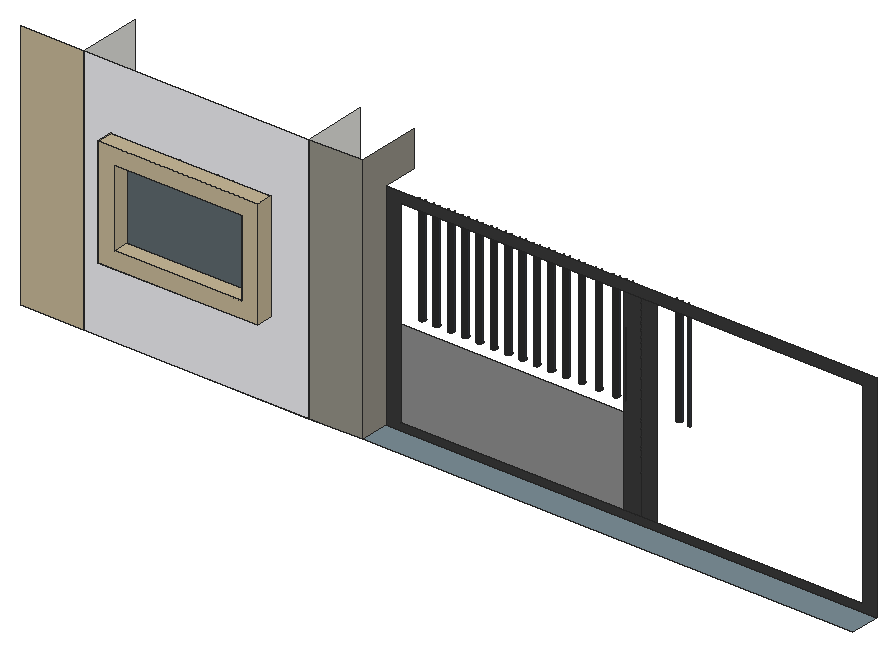
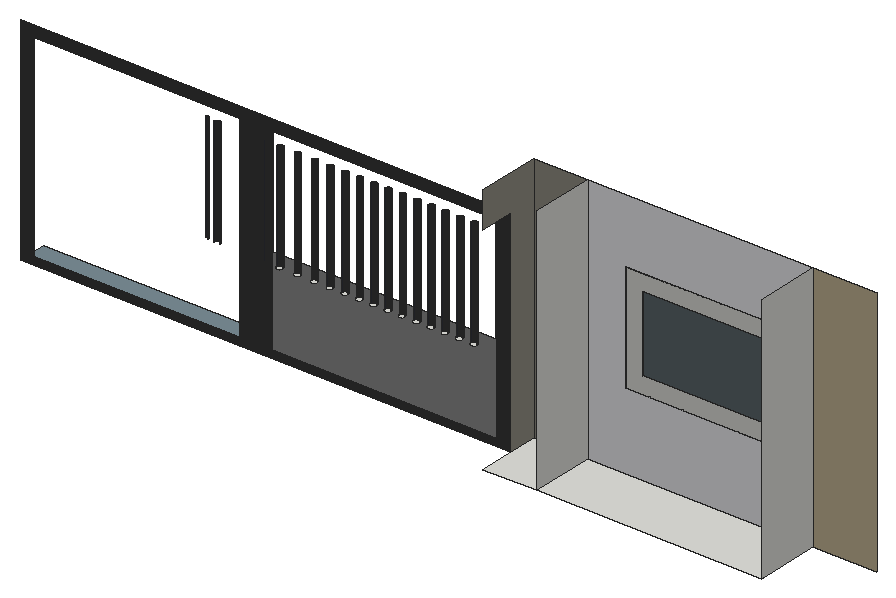
# SketchUp Ruby script. Lengths in inches.
U = 1.inch
M = Sketchup.active_model
def pt(a) = Geom::Point3d.new(a.map { |v| v * U })
def face(e, loops, mat)
  f = e.add_face(loops[0].map { |a| pt(a) })
  loops[1..].each { |l| e.add_face(l.map { |a| pt(a) }).erase! }
  f.material = f.back_material = mat if mat
  f
end
# faces: each face lists its corners as indices into pts; further lists are holes
def faces(e, pts, list, mat = nil) = list.each { |f| face(e, (f[0].is_a?(Array) ? f : [f]).map { |l| l.map { |i| pts[i] } }, mat) }
# xy, xz, yz: faces in a plane at the given z, y or x. An outline is a flat list of corners, or four numbers for a rectangle; further outlines are holes
def ring(l) = l.size == 4 ? [[l[0], l[1]], [l[2], l[1]], [l[2], l[3]], [l[0], l[3]]] : l.each_slice(2).to_a
def flat(e, list, mat, &to3) = list.each { |f| face(e, (f[0].is_a?(Array) ? f : [f]).map { |l| ring(l).map { |u, v| to3.(u, v) } }, mat) }
def xy(e, z, list, mat = nil) = flat(e, list, mat) { |x, y| [x, y, z] }
def xz(e, y, list, mat = nil) = flat(e, list, mat) { |x, z| [x, y, z] }
def yz(e, x, list, mat = nil) = flat(e, list, mat) { |y, z| [x, y, z] }
def lines(e, pts, list) = list.each { |a, b| e.add_line(pt(pts[a]), pt(pts[b])) }
# prism: a flat outline (further loops are holes) pulled along v
def prism(e, loops, v, mat = nil)
  f = face(e, loops, mat); d = Geom::Vector3d.new(v.map { |x| x * U })
  f.pushpull(f.normal.samedirection?(d) ? d.length : -d.length)
end
def box(e, o, s, mat = nil) = prism(e, [[o, [o[0] + s[0], o[1], o[2]], [o[0] + s[0], o[1] + s[1], o[2]], [o[0], o[1] + s[1], o[2]]]], [0, 0, s[2]], mat)
def at(x, y, z, deg = 0) = Geom::Transformation.translation(pt([x, y, z])) * Geom::Transformation.rotation(ORIGIN, Z_AXIS, deg.degrees)
def axes(o, x, y, z) = Geom::Transformation.new([*x, 0, *y, 0, *z, 0, *pt(o).to_a, 1])
def part(name) = M.definitions.add(name)
# library, detail: a bought-in or finely detailed component or shape, given as its bounding box
def library(name, o, s) = part(name).tap { |d| box(d.entities, o, s) }
def detail(e, o, s) = box(e.add_group.entities, o, s)
def put(e, d, t, mat = nil) = e.add_instance(d, t).tap { |i| i.material = mat if mat }
def group(e, t, mat = nil) = e.add_group.tap { |g| g.transformation = t; g.material = mat if mat }.entities
root = M.entities
M.materials.add("[Blinds Vertical Pattern]1").color = [239, 239, 242]
M.materials.add("[Color M04]").color = [142, 142, 142]
M.materials.add("[Color M07]").color = [58, 58, 58]
M.materials.add("[Formica Graystone]").color = [149, 146, 135]
M.materials.add("[Formica Laminate Dark]").color = [50, 53, 60]
M.materials.add("[Formica Speckled Grey]").color = [94, 105, 111]
M.materials.add("[Quartz Light Brown]").color = [199, 184, 152]
M.materials.add("[Square Glass Tile 01]").color = [123, 142, 151]
xy(root,0,[[14.76,96.24,66.82,111],[66.82,96.24,79.1,111]])
xy(root,0,[[79.1,96.24,192.64,102.91]],"[Square Glass Tile 01]")
xy(root,17.84,[[20.96,92.55,57.83,96.24]],"[Quartz Light Brown]")
xy(root,21.59,[[24.71,92.55,54.08,96.24]],"[Quartz Light Brown]")
xy(root,22.1875,[[84.71,106,84.53,106.02,84.36,106.09,84.22,106.2,84.11,106.34,84.04,106.51,84.02,106.6875,84.04,106.87,84.11,107.03,84.22,107.17,84.36,107.28,84.53,107.35,84.71,107.375,84.89,107.35,85.05,107.28,85.19,107.17,85.3,107.03,85.37,106.87,85.4,106.6875,85.37,106.51,85.3,106.34,85.19,106.2,85.05,106.09,84.89,106.02],[88.02,106,87.84,106.02,87.68,106.09,87.53,106.2,87.42,106.34,87.36,106.51,87.33,106.6875,87.36,106.87,87.42,107.03,87.53,107.17,87.68,107.28,87.84,107.35,88.02,107.375,88.2,107.35,88.36,107.28,88.51,107.17,88.62,107.03,88.68,106.87,88.71,106.6875,88.68,106.51,88.62,106.34,88.51,106.2,88.36,106.09,88.2,106.02],[91.33,106,91.15,106.02,90.99,106.09,90.85,106.2,90.74,106.34,90.67,106.51,90.65,106.6875,90.67,106.87,90.74,107.03,90.85,107.17,90.99,107.28,91.15,107.35,91.33,107.375,91.51,107.35,91.68,107.28,91.82,107.17,91.93,107.03,92,106.87,92.02,106.6875,92,106.51,91.93,106.34,91.82,106.2,91.68,106.09,91.51,106.02],[94.65,106,94.47,106.02,94.3,106.09,94.16,106.2,94.05,106.34,93.98,106.51,93.96,106.6875,93.98,106.87,94.05,107.03,94.16,107.17,94.3,107.28,94.47,107.35,94.65,107.375,94.82,107.35,94.99,107.28,95.13,107.17,95.24,107.03,95.31,106.87,95.33,106.6875,95.31,106.51,95.24,106.34,95.13,106.2,94.99,106.09,94.82,106.02],[97.96,106,97.78,106.02,97.61,106.09,97.47,106.2,97.36,106.34,97.29,106.51,97.27,106.6875,97.29,106.87,97.36,107.03,97.47,107.17,97.61,107.28,97.78,107.35,97.96,107.375,98.14,107.35,98.3,107.28,98.44,107.17,98.55,107.03,98.62,106.87,98.65,106.6875,98.62,106.51,98.55,106.34,98.44,106.2,98.3,106.09,98.14,106.02],
  [101.27,106,101.09,106.02,100.93,106.09,100.78,106.2,100.67,106.34,100.61,106.51,100.58,106.6875,100.61,106.87,100.67,107.03,100.78,107.17,100.93,107.28,101.09,107.35,101.27,107.375,101.45,107.35,101.61,107.28,101.76,107.17,101.87,107.03,101.93,106.87,101.96,106.6875,101.93,106.51,101.87,106.34,101.76,106.2,101.61,106.09,101.45,106.02],[104.58,106,104.4,106.02,104.24,106.09,104.1,106.2,103.99,106.34,103.92,106.51,103.9,106.6875,103.92,106.87,103.99,107.03,104.1,107.17,104.24,107.28,104.4,107.35,104.58,107.375,104.76,107.35,104.93,107.28,105.07,107.17,105.18,107.03,105.25,106.87,105.27,106.6875,105.25,106.51,105.18,106.34,105.07,106.2,104.93,106.09,104.76,106.02],[107.9,106,107.72,106.02,107.55,106.09,107.41,106.2,107.3,106.34,107.23,106.51,107.21,106.6875,107.23,106.87,107.3,107.03,107.41,107.17,107.55,107.28,107.72,107.35,107.9,107.375,108.07,107.35,108.24,107.28,108.38,107.17,108.49,107.03,108.56,106.87,108.58,106.6875,108.56,106.51,108.49,106.34,108.38,106.2,108.24,106.09,108.07,106.02],[111.21,106,111.03,106.02,110.86,106.09,110.72,106.2,110.61,106.34,110.54,106.51,110.52,106.6875,110.54,106.87,110.61,107.03,110.72,107.17,110.86,107.28,111.03,107.35,111.21,107.375,111.39,107.35,111.55,107.28,111.69,107.17,111.8,107.03,111.87,106.87,111.9,106.6875,111.87,106.51,111.8,106.34,111.69,106.2,111.55,106.09,111.39,106.02],[114.52,106,114.34,106.02,114.18,106.09,114.03,106.2,113.92,106.34,113.86,106.51,113.83,106.6875,113.86,106.87,113.92,107.03,114.03,107.17,114.18,107.28,114.34,107.35,114.52,107.375,114.7,107.35,114.86,107.28,115.01,107.17,115.12,107.03,115.18,106.87,115.21,106.6875,115.18,106.51,115.12,106.34,115.01,106.2,114.86,106.09,114.7,106.02],
  [117.96,106,117.78,106.02,117.61,106.09,117.47,106.2,117.36,106.34,117.29,106.51,117.27,106.6875,117.29,106.87,117.36,107.03,117.47,107.17,117.61,107.28,117.78,107.35,117.96,107.375,118.14,107.35,118.3,107.28,118.44,107.17,118.55,107.03,118.62,106.87,118.65,106.6875,118.62,106.51,118.55,106.34,118.44,106.2,118.3,106.09,118.14,106.02],[121.58,106,121.4,106.02,121.24,106.09,121.1,106.2,120.99,106.34,120.92,106.51,120.9,106.6875,120.92,106.87,120.99,107.03,121.1,107.17,121.24,107.28,121.4,107.35,121.58,107.375,121.76,107.35,121.93,107.28,122.07,107.17,122.18,107.03,122.25,106.87,122.27,106.6875,122.25,106.51,122.18,106.34,122.07,106.2,121.93,106.09,121.76,106.02],[125.52,106,125.34,106.02,125.18,106.09,125.03,106.2,124.92,106.34,124.86,106.51,124.83,106.6875,124.86,106.87,124.92,107.03,125.03,107.17,125.18,107.28,125.34,107.35,125.52,107.375,125.7,107.35,125.86,107.28,126.01,107.17,126.12,107.03,126.18,106.87,126.21,106.6875,126.18,106.51,126.12,106.34,126.01,106.2,125.86,106.09,125.7,106.02],[129.58,106,129.4,106.02,129.24,106.09,129.1,106.2,128.99,106.34,128.92,106.51,128.9,106.6875,128.92,106.87,128.99,107.03,129.1,107.17,129.24,107.28,129.4,107.35,129.58,107.375,129.76,107.35,129.93,107.28,130.07,107.17,130.18,107.03,130.25,106.87,130.27,106.6875,130.25,106.51,130.18,106.34,130.07,106.2,129.93,106.09,129.76,106.02]])
xy(root,39.28,[[24.71,92.55,54.08,96.24]],"[Quartz Light Brown]")
xy(root,43.03,[[20.96,92.55,57.83,96.24]],"[Quartz Light Brown]")
xz(root,92.55,[[[20.96,17.84,57.83,43.03],[24.71,21.59,54.08,39.28]]],"[Quartz Light Brown]")
xz(root,96.24,[[[20.96,17.84,57.83,43.03],[24.71,21.59,54.08,39.28]]])
xz(root,96.24,[[[14.76,0,66.82,57.8125],[20.96,17.84,57.83,43.03]]],"[Blinds Vertical Pattern]1")
xz(root,96.24,[[66.82,0,79.1,57.8125]],"[Formica Graystone]")
xz(root,96.24,[[24.71,21.59,54.08,39.28]],"[Formica Speckled Grey]")
xz(root,96.24,[[0,0,14.76,57.8125]],"[Quartz Light Brown]")
xz(root,102.91,[[82.65,1.75,134.27,22.1875]],"[Color M04]")
xz(root,102.91,[[[79.1,0,192.64,49.625],[82.65,1.75,189.5,47.21]],[134.27,1.75,138.0625,47.21],[138.0625,1.75,141.86,47.21]],"[Color M07]")
yz(root,14.76,[[96.24,0,111,57.8125]])
yz(root,20.96,[[92.55,17.84,96.24,43.03]],"[Quartz Light Brown]")
yz(root,24.71,[[92.55,21.59,96.24,39.28]],"[Quartz Light Brown]")
yz(root,54.08,[[92.55,21.59,96.24,39.28]],"[Quartz Light Brown]")
yz(root,57.83,[[92.55,17.84,96.24,43.03]],"[Quartz Light Brown]")
yz(root,66.82,[[96.24,0,111,57.8125]])
yz(root,79.1,[[96.24,0,102.91,0,102.91,49.625,111,49.625,111,57.8125,96.24,57.8125]],"[Formica Graystone]")
p = [[84.36,106.09,22.1875],[84.53,106.02,22.1875],[84.53,106.02,47.21],[84.36,106.09,47.21],[84.71,106,22.1875],[84.71,106,47.21],
  [84.89,106.02,22.1875],[84.89,106.02,47.21],[85.05,106.09,22.1875],[85.05,106.09,47.21],[87.68,106.09,22.1875],[87.84,106.02,22.1875],
  [87.84,106.02,47.21],[87.68,106.09,47.21],[88.02,106,22.1875],[88.02,106,47.21],[88.2,106.02,22.1875],[88.2,106.02,47.21],
  [88.36,106.09,22.1875],[88.36,106.09,47.21],[90.99,106.09,22.1875],[91.15,106.02,22.1875],[91.15,106.02,47.21],[90.99,106.09,47.21],
  [91.33,106,22.1875],[91.33,106,47.21],[91.51,106.02,22.1875],[91.51,106.02,47.21],[91.68,106.09,22.1875],[91.68,106.09,47.21],
  [94.3,106.09,22.1875],[94.47,106.02,22.1875],[94.47,106.02,47.21],[94.3,106.09,47.21],[94.65,106,22.1875],[94.65,106,47.21],
  [94.82,106.02,22.1875],[94.82,106.02,47.21],[94.99,106.09,22.1875],[94.99,106.09,47.21],[97.61,106.09,22.1875],[97.78,106.02,22.1875],
  [97.78,106.02,47.21],[97.61,106.09,47.21],[97.96,106,22.1875],[97.96,106,47.21],[98.14,106.02,22.1875],[98.14,106.02,47.21],
  [98.3,106.09,22.1875],[98.3,106.09,47.21],[100.93,106.09,22.1875],[101.09,106.02,22.1875],[101.09,106.02,47.21],[100.93,106.09,47.21],
  [101.27,106,22.1875],[101.27,106,47.21],[101.45,106.02,22.1875],[101.45,106.02,47.21],[101.61,106.09,22.1875],[101.61,106.09,47.21],
  [104.24,106.09,22.1875],[104.4,106.02,22.1875],[104.4,106.02,47.21],[104.24,106.09,47.21],[104.58,106,22.1875],[104.58,106,47.21],
  [104.76,106.02,22.1875],[104.76,106.02,47.21],[104.93,106.09,22.1875],[104.93,106.09,47.21],[107.55,106.09,22.1875],[107.72,106.02,22.1875],
  [107.72,106.02,47.21],[107.55,106.09,47.21],[107.9,106,22.1875],[107.9,106,47.21],[108.07,106.02,22.1875],[108.07,106.02,47.21],
  [108.24,106.09,22.1875],[108.24,106.09,47.21],[110.86,106.09,22.1875],[111.03,106.02,22.1875],[111.03,106.02,47.21],[110.86,106.09,47.21],
  [111.21,106,22.1875],[111.21,106,47.21],[111.39,106.02,22.1875],[111.39,106.02,47.21],[111.55,106.09,22.1875],[111.55,106.09,47.21],
  [114.18,106.09,22.1875],[114.34,106.02,22.1875],[114.34,106.02,47.21],[114.18,106.09,47.21],[114.52,106,22.1875],[114.52,106,47.21],
  [114.7,106.02,22.1875],[114.7,106.02,47.21],[114.86,106.09,22.1875],[114.86,106.09,47.21],[117.61,106.09,22.1875],[117.78,106.02,22.1875],
  [117.78,106.02,47.21],[117.61,106.09,47.21],[117.96,106,22.1875],[117.96,106,47.21],[118.14,106.02,22.1875],[118.14,106.02,47.21],
  [118.3,106.09,22.1875],[118.3,106.09,47.21],[121.24,106.09,22.1875],[121.4,106.02,22.1875],[121.4,106.02,47.21],[121.24,106.09,47.21],
  [121.58,106,22.1875],[121.58,106,47.21],[121.76,106.02,22.1875],[121.76,106.02,47.21],[121.93,106.09,22.1875],[121.93,106.09,47.21],
  [125.18,106.09,22.1875],[125.34,106.02,22.1875],[125.34,106.02,47.21],[125.18,106.09,47.21],[125.52,106,22.1875],[125.52,106,47.21],
  [125.7,106.02,22.1875],[125.7,106.02,47.21],[125.86,106.09,22.1875],[125.86,106.09,47.21],[129.24,106.09,22.1875],[129.4,106.02,22.1875],
  [129.4,106.02,47.21],[129.24,106.09,47.21],[129.58,106,22.1875],[129.58,106,47.21],[129.76,106.02,22.1875],[129.76,106.02,47.21],
  [129.93,106.09,22.1875],[129.93,106.09,47.21],[132.24,106.09,22.1875],[132.4,106.02,22.1875],[132.4,106.02,47.21],[132.24,106.09,47.21],
  [132.58,106,22.1875],[132.58,106,47.21],[132.76,106.02,22.1875],[132.76,106.02,47.21],[132.93,106.09,22.1875],[132.93,106.09,47.21],
  [143.74,106.09,22.1875],[143.9,106.02,22.1875],[143.9,106.02,47.21],[143.74,106.09,47.21],[144.08,106,22.1875],[144.08,106,47.21],
  [144.26,106.02,22.1875],[144.26,106.02,47.21],[144.43,106.09,22.1875],[144.43,106.09,47.21],[146.61,106.09,22.1875],[146.78,106.02,22.1875],
  [146.78,106.02,47.21],[146.61,106.09,47.21],[146.96,106,22.1875],[146.96,106,47.21],[147.14,106.02,22.1875],[147.14,106.02,47.21],
  [84.22,106.2,22.1875],[84.22,106.2,47.21],[85.19,106.2,22.1875],[85.19,106.2,47.21],[87.53,106.2,22.1875],[87.53,106.2,47.21],
  [88.51,106.2,22.1875],[88.51,106.2,47.21],[90.85,106.2,22.1875],[90.85,106.2,47.21],[91.82,106.2,22.1875],[91.82,106.2,47.21],
  [94.16,106.2,22.1875],[94.16,106.2,47.21],[95.13,106.2,22.1875],[95.13,106.2,47.21],[97.47,106.2,22.1875],[97.47,106.2,47.21],
  [98.44,106.2,22.1875],[98.44,106.2,47.21],[100.78,106.2,22.1875],[100.78,106.2,47.21],[101.76,106.2,22.1875],[101.76,106.2,47.21],
  [104.1,106.2,22.1875],[104.1,106.2,47.21],[105.07,106.2,22.1875],[105.07,106.2,47.21],[107.41,106.2,22.1875],[107.41,106.2,47.21],
  [108.38,106.2,22.1875],[108.38,106.2,47.21],[110.72,106.2,22.1875],[110.72,106.2,47.21],[111.69,106.2,22.1875],[111.69,106.2,47.21],
  [114.03,106.2,22.1875],[114.03,106.2,47.21],[115.01,106.2,22.1875],[115.01,106.2,47.21],[117.47,106.2,22.1875],[117.47,106.2,47.21],
  [118.44,106.2,22.1875],[118.44,106.2,47.21],[121.1,106.2,22.1875],[121.1,106.2,47.21],[122.07,106.2,22.1875],[122.07,106.2,47.21],
  [125.03,106.2,22.1875],[125.03,106.2,47.21],[126.01,106.2,22.1875],[126.01,106.2,47.21],[129.1,106.2,22.1875],[129.1,106.2,47.21],
  [130.07,106.2,22.1875],[130.07,106.2,47.21],[132.1,106.2,22.1875],[132.1,106.2,47.21],[133.07,106.2,22.1875],[133.07,106.2,47.21],
  [143.6,106.2,22.1875],[143.6,106.2,47.21],[144.57,106.2,22.1875],[144.57,106.2,47.21],[146.47,106.2,22.1875],[146.47,106.2,47.21],
  [84.11,106.34,22.1875],[84.11,106.34,47.21],[85.3,106.34,22.1875],[85.3,106.34,47.21],[87.42,106.34,22.1875],[87.42,106.34,47.21],
  [88.62,106.34,22.1875],[88.62,106.34,47.21],[90.74,106.34,22.1875],[90.74,106.34,47.21],[91.93,106.34,22.1875],[91.93,106.34,47.21],
  [94.05,106.34,22.1875],[94.05,106.34,47.21],[95.24,106.34,22.1875],[95.24,106.34,47.21],[97.36,106.34,22.1875],[97.36,106.34,47.21],
  [98.55,106.34,22.1875],[98.55,106.34,47.21],[100.67,106.34,22.1875],[100.67,106.34,47.21],[101.87,106.34,22.1875],[101.87,106.34,47.21],
  [103.99,106.34,22.1875],[103.99,106.34,47.21],[105.18,106.34,22.1875],[105.18,106.34,47.21],[107.3,106.34,22.1875],[107.3,106.34,47.21],
  [108.49,106.34,22.1875],[108.49,106.34,47.21],[110.61,106.34,22.1875],[110.61,106.34,47.21],[111.8,106.34,22.1875],[111.8,106.34,47.21],
  [113.92,106.34,22.1875],[113.92,106.34,47.21],[115.12,106.34,22.1875],[115.12,106.34,47.21],[117.36,106.34,22.1875],[117.36,106.34,47.21],
  [118.55,106.34,22.1875],[118.55,106.34,47.21],[120.99,106.34,22.1875],[120.99,106.34,47.21],[122.18,106.34,22.1875],[122.18,106.34,47.21],
  [124.92,106.34,22.1875],[124.92,106.34,47.21],[126.12,106.34,22.1875],[126.12,106.34,47.21],[128.99,106.34,22.1875],[128.99,106.34,47.21],
  [130.18,106.34,22.1875],[130.18,106.34,47.21],[131.99,106.34,22.1875],[131.99,106.34,47.21],[133.18,106.34,22.1875],[133.18,106.34,47.21],
  [143.49,106.34,22.1875],[143.49,106.34,47.21],[144.68,106.34,22.1875],[144.68,106.34,47.21],[146.36,106.34,22.1875],[146.36,106.34,47.21],
  [84.04,106.51,22.1875],[84.04,106.51,47.21],[85.37,106.51,22.1875],[85.37,106.51,47.21],[87.36,106.51,22.1875],[87.36,106.51,47.21],
  [88.68,106.51,22.1875],[88.68,106.51,47.21],[90.67,106.51,22.1875],[90.67,106.51,47.21],[92,106.51,22.1875],[92,106.51,47.21],
  [93.98,106.51,22.1875],[93.98,106.51,47.21],[95.31,106.51,22.1875],[95.31,106.51,47.21],[97.29,106.51,22.1875],[97.29,106.51,47.21],
  [98.62,106.51,22.1875],[98.62,106.51,47.21],[100.61,106.51,22.1875],[100.61,106.51,47.21],[101.93,106.51,22.1875],[101.93,106.51,47.21],
  [103.92,106.51,22.1875],[103.92,106.51,47.21],[105.25,106.51,22.1875],[105.25,106.51,47.21],[107.23,106.51,22.1875],[107.23,106.51,47.21],
  [108.56,106.51,22.1875],[108.56,106.51,47.21],[110.54,106.51,22.1875],[110.54,106.51,47.21],[111.87,106.51,22.1875],[111.87,106.51,47.21],
  [113.86,106.51,22.1875],[113.86,106.51,47.21],[115.18,106.51,22.1875],[115.18,106.51,47.21],[117.29,106.51,22.1875],[117.29,106.51,47.21],
  [118.62,106.51,22.1875],[118.62,106.51,47.21],[120.92,106.51,22.1875],[120.92,106.51,47.21],[122.25,106.51,22.1875],[122.25,106.51,47.21],
  [124.86,106.51,22.1875],[124.86,106.51,47.21],[126.18,106.51,22.1875],[126.18,106.51,47.21],[128.92,106.51,22.1875],[128.92,106.51,47.21],
  [130.25,106.51,22.1875],[130.25,106.51,47.21],[131.92,106.51,22.1875],[131.92,106.51,47.21],[133.25,106.51,22.1875],[133.25,106.51,47.21],
  [143.42,106.51,22.1875],[143.42,106.51,47.21],[144.75,106.51,22.1875],[144.75,106.51,47.21],[146.29,106.51,22.1875],[146.29,106.51,47.21],
  [84.02,106.6875,22.1875],[84.02,106.6875,47.21],[85.4,106.6875,22.1875],[85.4,106.6875,47.21],[87.33,106.6875,22.1875],[87.33,106.6875,47.21],
  [88.71,106.6875,22.1875],[88.71,106.6875,47.21],[90.65,106.6875,22.1875],[90.65,106.6875,47.21],[92.02,106.6875,22.1875],[92.02,106.6875,47.21],
  [93.96,106.6875,22.1875],[93.96,106.6875,47.21],[95.33,106.6875,22.1875],[95.33,106.6875,47.21],[97.27,106.6875,22.1875],[97.27,106.6875,47.21],
  [98.65,106.6875,22.1875],[98.65,106.6875,47.21],[100.58,106.6875,22.1875],[100.58,106.6875,47.21],[101.96,106.6875,22.1875],[101.96,106.6875,47.21],
  [103.9,106.6875,22.1875],[103.9,106.6875,47.21],[105.27,106.6875,22.1875],[105.27,106.6875,47.21],[107.21,106.6875,22.1875],[107.21,106.6875,47.21],
  [108.58,106.6875,22.1875],[108.58,106.6875,47.21],[110.52,106.6875,22.1875],[110.52,106.6875,47.21],[111.9,106.6875,22.1875],[111.9,106.6875,47.21],
  [113.83,106.6875,22.1875],[113.83,106.6875,47.21],[115.21,106.6875,22.1875],[115.21,106.6875,47.21],[117.27,106.6875,22.1875],[117.27,106.6875,47.21],
  [118.65,106.6875,22.1875],[118.65,106.6875,47.21],[120.9,106.6875,22.1875],[120.9,106.6875,47.21],[122.27,106.6875,22.1875],[122.27,106.6875,47.21],
  [124.83,106.6875,22.1875],[124.83,106.6875,47.21],[126.21,106.6875,22.1875],[126.21,106.6875,47.21],[128.9,106.6875,22.1875],[128.9,106.6875,47.21],
  [130.27,106.6875,22.1875],[130.27,106.6875,47.21],[131.9,106.6875,22.1875],[131.9,106.6875,47.21],[133.27,106.6875,22.1875],[133.27,106.6875,47.21],
  [143.4,106.6875,22.1875],[143.4,106.6875,47.21],[144.77,106.6875,22.1875],[144.77,106.6875,47.21],[146.27,106.6875,22.1875],[146.27,106.6875,47.21]]
faces(root,p,[[0,1,2,3],[1,4,5,2],[4,6,7,5],[6,8,9,7],[10,11,12,13],[11,14,15,12],[14,16,17,15],[16,18,19,17],
  [20,21,22,23],[21,24,25,22],[24,26,27,25],[26,28,29,27],[30,31,32,33],[31,34,35,32],[34,36,37,35],[36,38,39,37],
  [40,41,42,43],[41,44,45,42],[44,46,47,45],[46,48,49,47],[50,51,52,53],[51,54,55,52],[54,56,57,55],[56,58,59,57],
  [60,61,62,63],[61,64,65,62],[64,66,67,65],[66,68,69,67],[70,71,72,73],[71,74,75,72],[74,76,77,75],[76,78,79,77],
  [80,81,82,83],[81,84,85,82],[84,86,87,85],[86,88,89,87],[90,91,92,93],[91,94,95,92],[94,96,97,95],[96,98,99,97],
  [100,101,102,103],[101,104,105,102],[104,106,107,105],[106,108,109,107],[110,111,112,113],[111,114,115,112],[114,116,117,115],[116,118,119,117],
  [120,121,122,123],[121,124,125,122],[124,126,127,125],[126,128,129,127],[130,131,132,133],[131,134,135,132],[134,136,137,135],[136,138,139,137],
  [140,141,142,143],[141,144,145,142],[144,146,147,145],[146,148,149,147],[150,151,152,153],[151,154,155,152],[154,156,157,155],[156,158,159,157],
  [160,161,162,163],[161,164,165,162],[164,166,167,165],[168,0,3,169],[8,170,171,9],[172,10,13,173],[18,174,175,19],[176,20,23,177],
  [28,178,179,29],[180,30,33,181],[38,182,183,39],[184,40,43,185],[48,186,187,49],[188,50,53,189],[58,190,191,59],[192,60,63,193],
  [68,194,195,69],[196,70,73,197],[78,198,199,79],[200,80,83,201],[88,202,203,89],[204,90,93,205],[98,206,207,99],[208,100,103,209],
  [108,210,211,109],[212,110,113,213],[118,214,215,119],[216,120,123,217],[128,218,219,129],[220,130,133,221],[138,222,223,139],[224,140,143,225],
  [148,226,227,149],[228,150,153,229],[158,230,231,159],[232,160,163,233],[234,168,169,235],[170,236,237,171],[238,172,173,239],[174,240,241,175],
  [242,176,177,243],[178,244,245,179],[246,180,181,247],[182,248,249,183],[250,184,185,251],[186,252,253,187],[254,188,189,255],[190,256,257,191],
  [258,192,193,259],[194,260,261,195],[262,196,197,263],[198,264,265,199],[266,200,201,267],[202,268,269,203],[270,204,205,271],[206,272,273,207],
  [274,208,209,275],[210,276,277,211],[278,212,213,279],[214,280,281,215],[282,216,217,283],[218,284,285,219],[286,220,221,287],[222,288,289,223],
  [290,224,225,291],[226,292,293,227],[294,228,229,295],[230,296,297,231],[298,232,233,299],[300,234,235,301],[236,302,303,237],[304,238,239,305],
  [240,306,307,241],[308,242,243,309],[244,310,311,245],[312,246,247,313],[248,314,315,249],[316,250,251,317],[252,318,319,253],[320,254,255,321],
  [256,322,323,257],[324,258,259,325],[260,326,327,261],[328,262,263,329],[264,330,331,265],[332,266,267,333],[268,334,335,269],[336,270,271,337],
  [272,338,339,273],[340,274,275,341],[276,342,343,277],[344,278,279,345],[280,346,347,281],[348,282,283,349],[284,350,351,285],[352,286,287,353],
  [288,354,355,289],[356,290,291,357],[292,358,359,293],[360,294,295,361],[296,362,363,297],[364,298,299,365],[366,300,301,367],[302,368,369,303],
  [370,304,305,371],[306,372,373,307],[374,308,309,375],[310,376,377,311],[378,312,313,379],[314,380,381,315],[382,316,317,383],[318,384,385,319],
  [386,320,321,387],[322,388,389,323],[390,324,325,391],[326,392,393,327],[394,328,329,395],[330,396,397,331],[398,332,333,399],[334,400,401,335],
  [402,336,337,403],[338,404,405,339],[406,340,341,407],[342,408,409,343],[410,344,345,411],[346,412,413,347],[414,348,349,415],[350,416,417,351],
  [418,352,353,419],[354,420,421,355],[422,356,357,423],[358,424,425,359],[426,360,361,427],[362,428,429,363],[430,364,365,431]],"[Formica Laminate Dark]")
